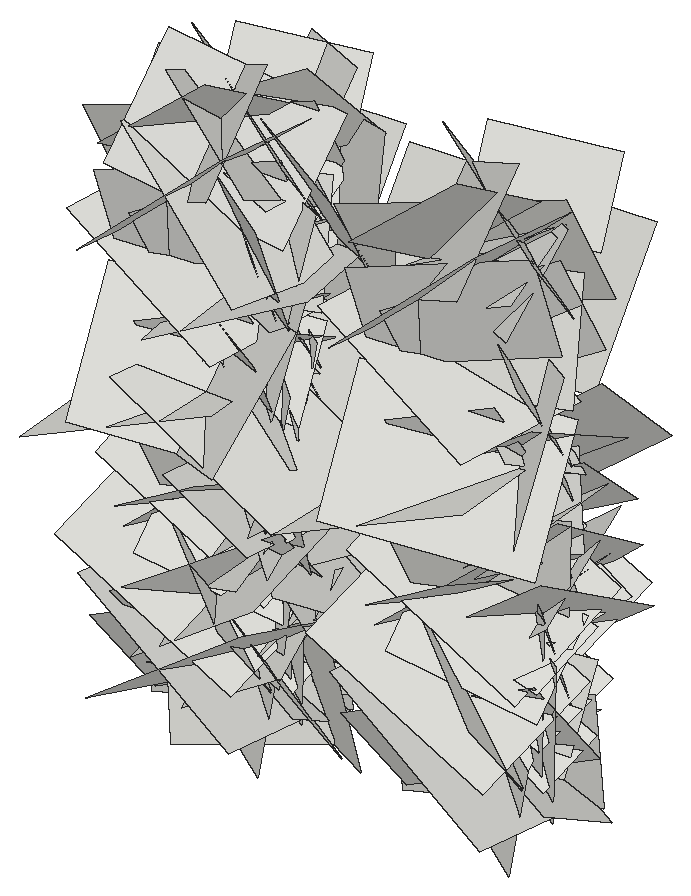
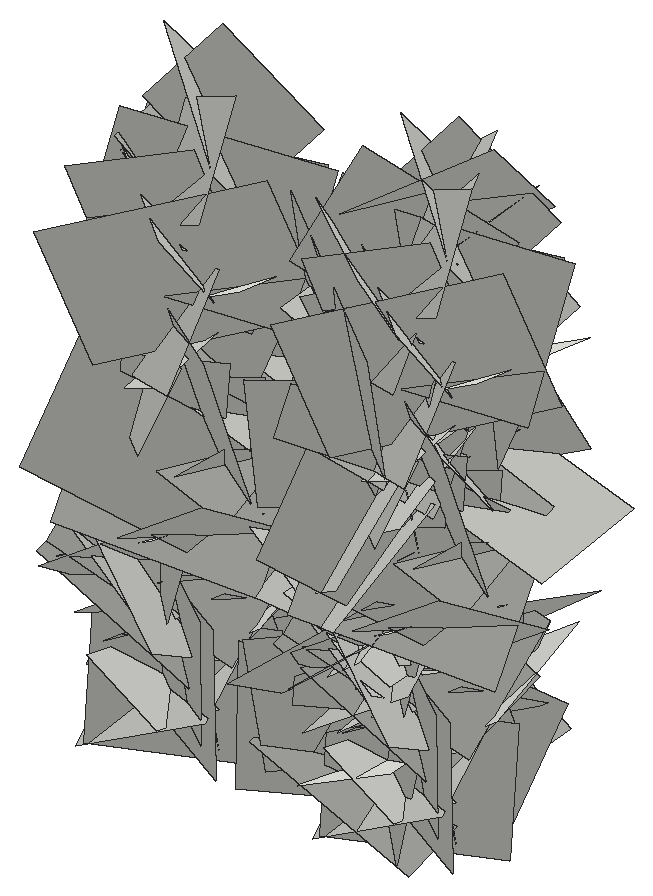
# SketchUp Ruby script. Lengths in inches.
U = 1.inch
M = Sketchup.active_model
def pt(a) = Geom::Point3d.new(a.map { |v| v * U })
def face(e, loops, mat)
  f = e.add_face(loops[0].map { |a| pt(a) })
  loops[1..].each { |l| e.add_face(l.map { |a| pt(a) }).erase! }
  f.material = f.back_material = mat if mat
  f
end
# faces: each face lists its corners as indices into pts; further lists are holes
def faces(e, pts, list, mat = nil) = list.each { |f| face(e, (f[0].is_a?(Array) ? f : [f]).map { |l| l.map { |i| pts[i] } }, mat) }
# xy, xz, yz: faces in a plane at the given z, y or x. An outline is a flat list of corners, or four numbers for a rectangle; further outlines are holes
def ring(l) = l.size == 4 ? [[l[0], l[1]], [l[2], l[1]], [l[2], l[3]], [l[0], l[3]]] : l.each_slice(2).to_a
def flat(e, list, mat, &to3) = list.each { |f| face(e, (f[0].is_a?(Array) ? f : [f]).map { |l| ring(l).map { |u, v| to3.(u, v) } }, mat) }
def xy(e, z, list, mat = nil) = flat(e, list, mat) { |x, y| [x, y, z] }
def xz(e, y, list, mat = nil) = flat(e, list, mat) { |x, z| [x, y, z] }
def yz(e, x, list, mat = nil) = flat(e, list, mat) { |y, z| [x, y, z] }
def lines(e, pts, list) = list.each { |a, b| e.add_line(pt(pts[a]), pt(pts[b])) }
# prism: a flat outline (further loops are holes) pulled along v
def prism(e, loops, v, mat = nil)
  f = face(e, loops, mat); d = Geom::Vector3d.new(v.map { |x| x * U })
  f.pushpull(f.normal.samedirection?(d) ? d.length : -d.length)
end
def box(e, o, s, mat = nil) = prism(e, [[o, [o[0] + s[0], o[1], o[2]], [o[0] + s[0], o[1] + s[1], o[2]], [o[0], o[1] + s[1], o[2]]]], [0, 0, s[2]], mat)
def at(x, y, z, deg = 0) = Geom::Transformation.translation(pt([x, y, z])) * Geom::Transformation.rotation(ORIGIN, Z_AXIS, deg.degrees)
def axes(o, x, y, z) = Geom::Transformation.new([*x, 0, *y, 0, *z, 0, *pt(o).to_a, 1])
def part(name) = M.definitions.add(name)
# library, detail: a bought-in or finely detailed component or shape, given as its bounding box
def library(name, o, s) = part(name).tap { |d| box(d.entities, o, s) }
def detail(e, o, s) = box(e.add_group.entities, o, s)
def put(e, d, t, mat = nil) = e.add_instance(d, t).tap { |i| i.material = mat if mat }
def group(e, t, mat = nil) = e.add_group.tap { |g| g.transformation = t; g.material = mat if mat }.entities
root = M.entities
c1 = part("Component\#6")
p = [[0.01,0,0],[0,3.24,4.54],[4.32,3.24,4.54],[4.33,0,0]]
faces(c1.entities,p,[[0,1,2,3]])
put(root,c1,axes([14.53,170.45,6.95],[-0.13562,-0.59571,0.16409],[0.06684,0.15411,0.60864],[0.65155,-0.13981,-0.02828]))
put(root,c1,axes([18.5,170.45,6.95],[0.13562,-0.59571,0.16409],[-0.06684,0.15411,0.60864],[-0.65155,-0.13981,-0.02828]))
put(root,c1,axes([24.34,170.45,6.95],[-0.13562,-0.59571,0.16409],[0.06684,0.15411,0.60864],[0.65155,-0.13981,-0.02828]))
put(root,c1,axes([18.5,172.51,13.7],[0.18405,-0.71312,-0.93832],[0.0125,-0.94735,0.72216],[-1.2492,-0.11455,-0.13102]))
put(root,c1,axes([14.53,172.51,13.7],[-0.18405,-0.71312,-0.93832],[-0.0125,-0.94735,0.72216],[1.2492,-0.11455,-0.13102]))
put(root,c1,axes([28.31,172.51,13.7],[0.18405,-0.71312,-0.93832],[0.0125,-0.94735,0.72216],[-1.2492,-0.11455,-0.13102]))
put(root,c1,axes([18.5,166.89,12.83],[-0.13197,1.26874,-0.04114],[-0.28106,-0.06642,-1.24587],[-1.31589,-0.11305,0.27023]))
put(root,c1,axes([14.53,166.89,12.83],[0.13197,1.26874,-0.04114],[0.28106,-0.06642,-1.24587],[1.31589,-0.11305,0.27023]))
put(root,c1,axes([28.31,166.89,12.83],[-0.13197,1.26874,-0.04114],[-0.28106,-0.06642,-1.24587],[-1.31589,-0.11305,0.27023]))
put(root,c1,axes([14.53,170.4375,18.81],[-0.19883,-0.70321,0.38228],[-0.06935,0.40479,0.71252],[0.84558,-0.13215,0.14832]))
put(root,c1,axes([18.5,170.4375,18.81],[0.19883,-0.70321,0.38228],[0.06935,0.40479,0.71252],[-0.84558,-0.13215,0.14832]))
put(root,c1,axes([24.34,170.4375,18.81],[-0.19883,-0.70321,0.38228],[-0.06935,0.40479,0.71252],[0.84558,-0.13215,0.14832]))
put(root,c1,axes([18.5,172.01,0.23],[0.18306,-1.21621,0.26629],[0.00588,0.26959,1.22768],[-1.31971,-0.16751,0.04241]))
put(root,c1,axes([14.53,172.01,0.23],[-0.18306,-1.21621,0.26629],[-0.00588,0.26959,1.22768],[1.31971,-0.16751,0.04241]))
put(root,c1,axes([28.31,172.01,0.23],[0.18306,-1.21621,0.26629],[0.00588,0.26959,1.22768],[-1.31971,-0.16751,0.04241]))
put(root,c1,axes([18.5,167.43,21.54],[-0.05686,1.16606,-0.16138],[0.18622,-0.15181,-1.15529],[-1.23383,-0.07665,-0.16693]))
put(root,c1,axes([14.53,167.43,21.54],[0.05686,1.16606,-0.16138],[-0.18622,-0.15181,-1.15529],[1.23383,-0.07665,-0.16693]))
put(root,c1,axes([28.31,167.43,21.54],[-0.05686,1.16606,-0.16138],[0.18622,-0.15181,-1.15529],[-1.23383,-0.07665,-0.16693]))
put(root,c1,axes([18.5,170.29,20.28],[-0.01759,0.35165,-0.94572],[-0.09141,-0.94289,-0.34909],[-1.06561,0.07508,0.04555]))
put(root,c1,axes([14.53,170.29,20.28],[0.01759,0.35165,-0.94572],[0.09141,-0.94289,-0.34909],[1.06561,0.07508,0.04555]))
put(root,c1,axes([28.31,170.29,20.28],[-0.01759,0.35165,-0.94572],[-0.09141,-0.94289,-0.34909],[-1.06561,0.07508,0.04555]))
put(root,c1,axes([18.5,166.61,20.4],[-0.01588,0.7114,0.79833],[0.18087,0.78977,-0.70057],[-1.11894,0.11757,-0.12458]))
put(root,c1,axes([14.53,166.61,20.4],[0.01588,0.7114,0.79833],[-0.18087,0.78977,-0.70057],[1.11894,0.11757,-0.12458]))
put(root,c1,axes([28.31,166.61,20.4],[-0.01588,0.7114,0.79833],[0.18087,0.78977,-0.70057],[-1.11894,0.11757,-0.12458]))
put(root,c1,axes([14.53,169.875,11.58],[-0.08121,-0.31714,0.54408],[0.11401,0.53345,0.32609],[0.65774,-0.13162,0.01065]))
put(root,c1,axes([18.5,169.875,11.58],[0.08121,-0.31714,0.54408],[-0.11401,0.53345,0.32609],[-0.65774,-0.13162,0.01065]))
put(root,c1,axes([24.34,169.875,11.58],[-0.08121,-0.31714,0.54408],[0.11401,0.53345,0.32609],[0.65774,-0.13162,0.01065]))
put(root,c1,axes([18.5,169.82,1.95],[0.02915,-0.64251,0.76006],[0.08177,0.75943,0.6392],[-1.05178,0.04123,0.07076]))
put(root,c1,axes([14.53,169.82,1.95],[-0.02915,-0.64251,0.76006],[-0.08177,0.75943,0.6392],[1.05178,0.04123,0.07076]))
put(root,c1,axes([28.31,169.82,1.95],[0.02915,-0.64251,0.76006],[0.08177,0.75943,0.6392],[-1.05178,0.04123,0.07076]))
put(root,c1,axes([18.5,173.1,4.27],[-0.006,-1.20261,-0.38975],[0.07836,-0.3894,1.20046],[-1.33775,-0.01742,0.07206]))
put(root,c1,axes([14.53,173.1,4.27],[0.006,-1.20261,-0.38975],[-0.07836,-0.3894,1.20046],[1.33775,-0.01742,0.07206]))
put(root,c1,axes([28.31,173.1,4.27],[-0.006,-1.20261,-0.38975],[0.07836,-0.3894,1.20046],[-1.33775,-0.01742,0.07206]))
put(root,c1,axes([14.53,169.57,7.53],[0.02893,-0.34038,0.60393],[-0.06424,0.60091,0.34142],[0.73203,0.06619,0.00609]))
put(root,c1,axes([18.5,169.57,7.53],[-0.02893,-0.34038,0.60393],[0.06424,0.60091,0.34142],[-0.73203,0.06619,0.00609]))
put(root,c1,axes([24.34,169.57,7.53],[0.02893,-0.34038,0.60393],[-0.06424,0.60091,0.34142],[0.73203,0.06619,0.00609]))
put(root,c1,axes([18.5,172.68,14.25],[-0.15371,-1.16437,-0.05617],[-0.14183,-0.0396,1.1664],[-1.22751,0.15038,-0.12774]))
put(root,c1,axes([14.53,172.68,14.25],[0.15371,-1.16437,-0.05617],[0.14183,-0.0396,1.1664],[1.22751,0.15038,-0.12774]))
put(root,c1,axes([28.31,172.68,14.25],[-0.15371,-1.16437,-0.05617],[-0.14183,-0.0396,1.1664],[-1.22751,0.15038,-0.12774]))
put(root,c1,axes([18.5,172.08,18.68],[0.05145,-0.65016,0.07549],[-0.09383,0.06848,0.64671],[-0.68743,-0.05801,-0.08262]))
put(root,c1,axes([14.53,172.08,18.68],[-0.05145,-0.65016,0.07549],[0.09383,0.06848,0.64671],[0.68743,-0.05801,-0.08262]))
put(root,c1,axes([24.34,172.08,18.68],[-0.05145,-0.65016,0.07549],[0.09383,0.06848,0.64671],[0.68743,-0.05801,-0.08262]))
put(root,c1,axes([14.53,168.08,6.15],[-0.10311,0.69666,0.5447],[-0.01855,0.54636,-0.70191],[0.9372,0.08746,0.04604]))
put(root,c1,axes([18.5,168.08,6.15],[0.10311,0.69666,0.5447],[0.01855,0.54636,-0.70191],[-0.9372,0.08746,0.04604]))
put(root,c1,axes([24.34,168.08,6.15],[-0.10311,0.69666,0.5447],[-0.01855,0.54636,-0.70191],[0.9372,0.08746,0.04604]))
put(root,c1,axes([18.5,170.37,5.28],[0.04044,0.69271,-0.86885],[-0.14808,-0.85947,-0.69137],[-1.16852,0.13289,0.05755]))
put(root,c1,axes([14.53,170.37,5.28],[-0.04044,0.69271,-0.86885],[0.14808,-0.85947,-0.69137],[1.16852,0.13289,0.05755]))
put(root,c1,axes([28.31,170.37,5.28],[0.04044,0.69271,-0.86885],[-0.14808,-0.85947,-0.69137],[-1.16852,0.13289,0.05755]))
put(root,c1,axes([18.5,171.61,19.65],[0.05512,0.44879,-0.89687],[0.12411,-0.89465,-0.44089],[-1.05579,-0.08174,-0.09865]))
put(root,c1,axes([14.53,171.61,19.65],[-0.05512,0.44879,-0.89687],[-0.12411,-0.89465,-0.44089],[1.05579,-0.08174,-0.09865]))
put(root,c1,axes([28.31,171.61,19.65],[0.05512,0.44879,-0.89687],[0.12411,-0.89465,-0.44089],[-1.05579,-0.08174,-0.09865]))
put(root,c1,axes([18.5,172.8125,18.6875],[0.10377,-0.25363,-0.96814],[-0.17625,-0.96337,0.23557],[-1.04612,0.13715,-0.13572]))
put(root,c1,axes([14.53,172.8125,18.6875],[-0.10377,-0.25363,-0.96814],[0.17625,-0.96337,0.23557],[1.04612,0.13715,-0.13572]))
put(root,c1,axes([28.31,172.8125,18.6875],[0.10377,-0.25363,-0.96814],[-0.17625,-0.96337,0.23557],[-1.04612,0.13715,-0.13572]))
put(root,c1,axes([18.5,173.43,2.26],[-0.13173,-0.86629,-0.47025],[0.00519,-0.47451,0.87284],[-1.04483,0.10686,0.06363]))
put(root,c1,axes([14.53,173.43,2.26],[0.13173,-0.86629,-0.47025],[-0.00519,-0.47451,0.87284],[1.04483,0.10686,0.06363]))
put(root,c1,axes([28.31,173.43,2.26],[-0.13173,-0.86629,-0.47025],[0.00519,-0.47451,0.87284],[-1.04483,0.10686,0.06363]))
put(root,c1,axes([14.53,172.62,2.82],[-0.11022,-0.07985,-0.84847],[0.01268,-0.85481,0.07898],[0.90326,0.00226,-0.10464]))
put(root,c1,axes([18.5,172.62,2.82],[0.11022,-0.07985,-0.84847],[-0.01268,-0.85481,0.07898],[-0.90326,0.00226,-0.10464]))
put(root,c1,axes([24.34,172.62,2.82],[-0.11022,-0.07985,-0.84847],[0.01268,-0.85481,0.07898],[0.90326,0.00226,-0.10464]))
put(root,c1,axes([18.5,172.18,10.26],[-0.13568,0.14362,-0.9313],[-0.0793,-0.93844,-0.13444],[-0.9957,0.05517,0.13761]))
put(root,c1,axes([28.31,172.18,10.26],[-0.13568,0.14362,-0.9313],[-0.0793,-0.93844,-0.13444],[-0.9957,0.05517,0.13761]))
put(root,c1,axes([14.53,172.18,10.26],[0.13568,0.14362,-0.9313],[0.0793,-0.93844,-0.13444],[0.9957,0.05517,0.13761]))
put(root,c1,axes([14.53,169.25,3.37],[-0.12984,0.58451,0.34416],[-0.01188,0.34794,-0.59491],[0.71891,0.11132,0.05233]))
put(root,c1,axes([18.5,169.25,3.37],[0.12984,0.58451,0.34416],[0.01188,0.34794,-0.59491],[-0.71891,0.11132,0.05233]))
put(root,c1,axes([24.34,169.25,3.37],[-0.12984,0.58451,0.34416],[-0.01188,0.34794,-0.59491],[0.71891,0.11132,0.05233]))
put(root,c1,axes([18.5,174.625,6.88],[-0.07025,-1.10898,-0.49527],[0.16839,-0.49966,1.09755],[-1.27636,-0.00489,0.17206]))
put(root,c1,axes([14.53,174.625,6.88],[0.07025,-1.10898,-0.49527],[-0.16839,-0.49966,1.09755],[1.27636,-0.00489,0.17206]))
put(root,c1,axes([28.31,174.625,6.88],[-0.07025,-1.10898,-0.49527],[0.16839,-0.49966,1.09755],[-1.27636,-0.00489,0.17206]))
put(root,c1,axes([18.5,173.47,4.9],[-0.07332,-0.2848,-0.87141],[0.0336,-0.87411,0.28317],[-0.9712,-0.00874,0.07558]))
put(root,c1,axes([14.53,173.47,4.9],[0.07332,-0.2848,-0.87141],[-0.0336,-0.87411,0.28317],[0.9712,-0.00874,0.07558]))
put(root,c1,axes([28.31,173.47,4.9],[-0.07332,-0.2848,-0.87141],[0.0336,-0.87411,0.28317],[-0.9712,-0.00874,0.07558]))
put(root,c1,axes([14.53,169.67,8.54],[-0.12628,0.08221,0.86907],[-0.11161,0.86937,-0.09667],[0.91857,0.11693,0.10773]))
put(root,c1,axes([18.5,169.67,8.54],[0.12628,0.08221,0.86907],[0.11161,0.86937,-0.09667],[-0.91857,0.11693,0.10773]))
put(root,c1,axes([24.34,169.67,8.54],[-0.12628,0.08221,0.86907],[-0.11161,0.86937,-0.09667],[0.91857,0.11693,0.10773]))
put(root,c1,axes([14.53,173.61,18.42],[0.00387,-0.64214,-0.38262],[0.01033,-0.38255,0.64212],[0.79227,0.00812,-0.0065]))
put(root,c1,axes([18.5,173.61,18.42],[-0.00387,-0.64214,-0.38262],[-0.01033,-0.38255,0.64212],[-0.79227,0.00812,-0.0065]))
put(root,c1,axes([24.34,173.61,18.42],[0.00387,-0.64214,-0.38262],[0.01033,-0.38255,0.64212],[0.79227,0.00812,-0.0065]))
put(root,c1,axes([18.5,173.47,6.03],[0.02519,-0.71274,-0.22366],[-0.1783,-0.22314,0.69319],[-0.7715,0.02829,-0.1675]))
put(root,c1,axes([14.53,173.47,6.03],[-0.02519,-0.71274,-0.22366],[0.1783,-0.22314,0.69319],[0.7715,0.02829,-0.1675]))
put(root,c1,axes([28.31,173.47,6.03],[0.02519,-0.71274,-0.22366],[-0.1783,-0.22314,0.69319],[-0.7715,0.02829,-0.1675]))
put(root,c1,axes([18.5,170.23,14.27],[0.02775,1.05616,-0.50439],[0.01222,-0.50473,-1.05626],[-1.24058,0.01865,-0.02169]))
put(root,c1,axes([14.53,170.23,14.27],[-0.02775,1.05616,-0.50439],[-0.01222,-0.50473,-1.05626],[1.24058,0.01865,-0.02169]))
put(root,c1,axes([28.31,170.23,14.27],[0.02775,1.05616,-0.50439],[0.01222,-0.50473,-1.05626],[-1.24058,0.01865,-0.02169]))
put(root,c1,axes([18.5,172.3,17.31],[0.17712,-0.66279,0.75583],[-0.05377,0.75967,0.67737],[-1.06423,-0.14869,0.09157]))
put(root,c1,axes([14.53,172.3,17.31],[-0.17712,-0.66279,0.75583],[0.05377,0.75967,0.67737],[1.06423,-0.14869,0.09157]))
put(root,c1,axes([28.31,172.3,17.31],[0.17712,-0.66279,0.75583],[-0.05377,0.75967,0.67737],[-1.06423,-0.14869,0.09157]))
put(root,c1,axes([18.5,171.9,21.66],[-0.05821,0.63814,-1.10333],[-0.23209,-1.09266,-0.62107],[-1.33097,0.16262,0.15656]))
put(root,c1,axes([14.53,171.9,21.66],[0.05821,0.63814,-1.10333],[0.23209,-1.09266,-0.62107],[1.33097,0.16262,0.15656]))
put(root,c1,axes([28.31,171.9,21.66],[-0.05821,0.63814,-1.10333],[-0.23209,-1.09266,-0.62107],[-1.33097,0.16262,0.15656]))
put(root,c1,axes([14.53,171.64,6.09],[-0.04085,-0.22846,0.61977],[0.06336,0.61707,0.23119],[0.6973,-0.06945,0.0153]))
put(root,c1,axes([18.5,171.64,6.09],[0.04085,-0.22846,0.61977],[-0.06336,0.61707,0.23119],[-0.6973,-0.06945,0.0153]))
put(root,c1,axes([24.34,171.64,6.09],[-0.04085,-0.22846,0.61977],[0.06336,0.61707,0.23119],[0.6973,-0.06945,0.0153]))
put(root,c1,axes([18.5,170.14,10.52],[-0.06349,0.95893,0.01002],[0.03302,0.01198,-0.96028],[-1.01599,-0.05954,-0.03183]))
put(root,c1,axes([14.53,170.14,10.52],[0.06349,0.95893,0.01002],[-0.03302,0.01198,-0.96028],[1.01599,-0.05954,-0.03183]))
put(root,c1,axes([28.31,170.14,10.52],[-0.06349,0.95893,0.01002],[0.03302,0.01198,-0.96028],[-1.01599,-0.05954,-0.03183]))
put(root,c1,axes([14.53,174.87,19.3],[-0.1513,-0.51657,-0.73784],[-0.06675,-0.7395,0.52991],[0.9524,-0.13389,-0.08008]))
put(root,c1,axes([18.5,174.87,19.3],[0.1513,-0.51657,-0.73784],[0.06675,-0.7395,0.52991],[-0.9524,-0.13389,-0.08008]))
put(root,c1,axes([24.34,174.87,19.3],[-0.1513,-0.51657,-0.73784],[-0.06675,-0.7395,0.52991],[0.9524,-0.13389,-0.08008]))
put(root,c1,axes([18.5,172.92,11.6],[-0.15777,-0.72106,0.34948],[0.01112,0.35368,0.73418],[-0.84929,0.13857,-0.05531]))
put(root,c1,axes([14.53,172.92,11.6],[0.15777,-0.72106,0.34948],[-0.01112,0.35368,0.73418],[0.84929,0.13857,-0.05531]))
put(root,c1,axes([28.31,172.92,11.6],[-0.15777,-0.72106,0.34948],[0.01112,0.35368,0.73418],[-0.84929,0.13857,-0.05531]))
put(root,c1,axes([18.5,169.35,10.4],[0.15861,0.37048,1.309],[-0.06067,1.31744,-0.36632],[-1.44077,-0.01469,0.15953]))
put(root,c1,axes([14.53,169.35,10.4],[-0.15861,0.37048,1.309],[0.06067,1.31744,-0.36632],[1.44077,-0.01469,0.15953]))
put(root,c1,axes([28.31,169.35,10.4],[0.15861,0.37048,1.309],[-0.06067,1.31744,-0.36632],[-1.44077,-0.01469,0.15953]))
put(root,c1,axes([18.5,171.5,10.51],[-0.09816,1.08592,-0.68794],[0.27584,-0.65961,-1.07622],[-1.33441,-0.21623,-0.17187]))
put(root,c1,axes([14.53,171.5,10.51],[0.09816,1.08592,-0.68794],[-0.27584,-0.65961,-1.07622],[1.33441,-0.21623,-0.17187]))
put(root,c1,axes([28.31,171.5,10.51],[-0.09816,1.08592,-0.68794],[0.27584,-0.65961,-1.07622],[-1.33441,-0.21623,-0.17187]))
put(root,c1,axes([18.5,170.67,8.7],[0.18467,1.04701,-0.56036],[0.0341,-0.57031,-1.0556],[-1.25832,0.1382,-0.11085]))
put(root,c1,axes([14.53,170.67,8.7],[-0.18467,1.04701,-0.56036],[-0.0341,-0.57031,-1.0556],[1.25832,0.1382,-0.11085]))
put(root,c1,axes([28.31,170.67,8.7],[0.18467,1.04701,-0.56036],[0.0341,-0.57031,-1.0556],[-1.25832,0.1382,-0.11085]))
put(root,c1,axes([18.5,174.22,3.89],[-0.08779,-0.72671,-0.31501],[-0.02258,-0.31457,0.73129],[-0.83927,0.08448,0.01327]))
put(root,c1,axes([14.53,174.22,3.89],[0.08779,-0.72671,-0.31501],[0.02258,-0.31457,0.73129],[0.83927,0.08448,0.01327]))
put(root,c1,axes([28.31,174.22,3.89],[-0.08779,-0.72671,-0.31501],[-0.02258,-0.31457,0.73129],[-0.83927,0.08448,0.01327]))
put(root,c1,axes([18.5,174.19,-1.125],[0.19779,-1.01545,0.55728],[-0.13113,0.54376,1.03224],[-1.22079,-0.22293,-0.02059]))
put(root,c1,axes([14.53,174.19,-1.125],[-0.19779,-1.01545,0.55728],[0.13113,0.54376,1.03224],[1.22079,-0.22293,-0.02059]))
put(root,c1,axes([28.31,174.19,-1.125],[0.19779,-1.01545,0.55728],[-0.13113,0.54376,1.03224],[-1.22079,-0.22293,-0.02059]))
put(root,c1,axes([14.53,171.41,10.85],[-0.07762,0.04197,0.59758],[0.0194,0.6019,-0.04003],[0.6347,-0.01326,0.07431]))
put(root,c1,axes([18.5,171.41,10.85],[0.07762,0.04197,0.59758],[-0.0194,0.6019,-0.04003],[-0.6347,-0.01326,0.07431]))
put(root,c1,axes([24.34,171.41,10.85],[-0.07762,0.04197,0.59758],[0.0194,0.6019,-0.04003],[0.6347,-0.01326,0.07431]))
put(root,c1,axes([18.5,173.32,3.72],[-0.0912,0.22313,-1.04907],[-0.17676,-1.04242,-0.20804],[-1.12306,0.14594,0.11794]))
put(root,c1,axes([14.53,173.32,3.72],[0.0912,0.22313,-1.04907],[0.17676,-1.04242,-0.20804],[1.12306,0.14594,0.11794]))
put(root,c1,axes([28.31,173.32,3.72],[-0.0912,0.22313,-1.04907],[-0.17676,-1.04242,-0.20804],[-1.12306,0.14594,0.11794]))
put(root,c1,axes([14.53,173.27,2.31],[0.02745,-0.60704,0.2793],[-0.09658,0.2737,0.6033],[0.70169,0.06142,0.07211]))
put(root,c1,axes([18.5,173.27,2.31],[-0.02745,-0.60704,0.2793],[0.09658,0.2737,0.6033],[-0.70169,0.06142,0.07211]))
put(root,c1,axes([24.34,173.27,2.31],[0.02745,-0.60704,0.2793],[-0.09658,0.2737,0.6033],[0.70169,0.06142,0.07211]))
put(root,c1,axes([18.5,172.23,12.17],[-0.04321,-0.56467,0.8488],[0.06772,0.84639,0.56613],[-1.07851,0.07577,0.00154]))
put(root,c1,axes([14.53,172.23,12.17],[0.04321,-0.56467,0.8488],[-0.06772,0.84639,0.56613],[1.07851,0.07577,0.00154]))
put(root,c1,axes([28.31,172.23,12.17],[-0.04321,-0.56467,0.8488],[0.06772,0.84639,0.56613],[-1.07851,0.07577,0.00154]))
put(root,c1,axes([18.5,170.77,1.94],[-0.10305,0.14958,1.1623],[0.03,1.16625,-0.14772],[-1.24184,0.01576,-0.10002]))
put(root,c1,axes([14.53,170.77,1.94],[0.10305,0.14958,1.1623],[-0.03,1.16625,-0.14772],[1.24184,0.01576,-0.10002]))
put(root,c1,axes([28.31,170.77,1.94],[-0.10305,0.14958,1.1623],[0.03,1.16625,-0.14772],[-1.24184,0.01576,-0.10002]))
put(root,c1,axes([18.5,172.28,10.96],[-0.19399,-0.26613,0.68464],[0.06344,0.69782,0.28725],[-0.77602,0.12358,-0.14766]))
put(root,c1,axes([14.53,172.28,10.96],[0.19399,-0.26613,0.68464],[-0.06344,0.69782,0.28725],[0.77602,0.12358,-0.14766]))
put(root,c1,axes([28.31,172.28,10.96],[-0.19399,-0.26613,0.68464],[0.06344,0.69782,0.28725],[-0.77602,0.12358,-0.14766]))
put(root,c1,axes([18.5,172.17,3.88],[-0.10658,-0.21665,0.83392],[0.00523,0.83942,0.21867],[-0.91328,0.03009,-0.09606]))
put(root,c1,axes([14.53,172.17,3.88],[0.10658,-0.21665,0.83392],[-0.00523,0.83942,0.21867],[0.91328,0.03009,-0.09606]))
put(root,c1,axes([28.31,172.17,3.88],[-0.10658,-0.21665,0.83392],[0.00523,0.83942,0.21867],[-0.91328,0.03009,-0.09606]))
put(root,c1,axes([18.5,172.79,12.08],[-0.24348,0.91998,-0.78066],[-0.03668,-0.79938,-0.93185],[-1.27843,-0.15228,0.17542]))
put(root,c1,axes([14.53,172.79,12.08],[0.24348,0.91998,-0.78066],[0.03668,-0.79938,-0.93185],[1.27843,-0.15228,0.17542]))
put(root,c1,axes([28.31,172.79,12.08],[-0.24348,0.91998,-0.78066],[-0.03668,-0.79938,-0.93185],[-1.27843,-0.15228,0.17542]))
put(root,c1,axes([18.5,171.28,0.09],[0.0277,-0.00252,1.28462],[-0.09278,1.2819,0.0043],[-1.35854,-0.08759,0.0259]))
put(root,c1,axes([28.31,171.28,0.09],[0.0277,-0.00252,1.28462],[-0.09278,1.2819,0.0043],[-1.35854,-0.08759,0.0259]))
put(root,c1,axes([14.53,171.28,0.09],[-0.0277,-0.00252,1.28462],[0.09278,1.2819,0.0043],[1.35854,-0.08759,0.0259]))
put(root,c1,axes([14.53,174.97,1.18],[-0.10067,-0.62121,-0.06126],[0.13552,-0.08001,0.61313],[0.64765,-0.07982,-0.13782]))
put(root,c1,axes([18.5,174.97,1.18],[0.10067,-0.62121,-0.06126],[-0.13552,-0.08001,0.61313],[-0.64765,-0.07982,-0.13782]))
put(root,c1,axes([24.34,174.97,1.18],[-0.10067,-0.62121,-0.06126],[0.13552,-0.08001,0.61313],[0.64765,-0.07982,-0.13782]))
put(root,c1,axes([18.5,176.36,18.92],[-0.19548,-0.4632,-1.27504],[0.04093,-1.28804,0.46234],[-1.43738,0.02631,0.18657]))
put(root,c1,axes([14.53,176.36,18.92],[0.19548,-0.4632,-1.27504],[-0.04093,-1.28804,0.46234],[1.43738,0.02631,0.18657]))
put(root,c1,axes([28.31,176.36,18.92],[-0.19548,-0.4632,-1.27504],[0.04093,-1.28804,0.46234],[-1.43738,0.02631,0.18657]))
put(root,c1,axes([18.5,176.11,6.43],[-0.23133,-1.0261,-0.61864],[-0.04368,-0.62202,1.04624],[-1.2693,0.20842,0.07674]))
put(root,c1,axes([14.53,176.11,6.43],[0.23133,-1.0261,-0.61864],[0.04368,-0.62202,1.04624],[1.2693,0.20842,0.07674]))
put(root,c1,axes([28.31,176.11,6.43],[-0.23133,-1.0261,-0.61864],[-0.04368,-0.62202,1.04624],[-1.2693,0.20842,0.07674]))
put(root,c1,axes([18.5,175.17,6.35],[-0.11089,-0.78923,-0.08985],[-0.10937,-0.07636,0.79084],[-0.83485,0.11483,-0.09167]))
put(root,c1,axes([14.53,175.17,6.35],[0.11089,-0.78923,-0.08985],[0.10937,-0.07636,0.79084],[0.83485,0.11483,-0.09167]))
put(root,c1,axes([28.31,175.17,6.35],[-0.11089,-0.78923,-0.08985],[-0.10937,-0.07636,0.79084],[-0.83485,0.11483,-0.09167]))
put(root,c1,axes([14.53,175.4,4.97],[0.01432,-0.74639,-0.04739],[-0.08616,-0.04858,0.74199],[0.78807,0.00825,0.08199]))
put(root,c1,axes([18.5,175.4,4.97],[-0.01432,-0.74639,-0.04739],[0.08616,-0.04858,0.74199],[-0.78807,0.00825,0.08199]))
put(root,c1,axes([24.34,175.4,4.97],[0.01432,-0.74639,-0.04739],[-0.08616,-0.04858,0.74199],[0.78807,0.00825,0.08199]))
put(root,c1,axes([18.5,173.68,14.42],[-0.07839,0.88361,-0.83437],[0.27617,-0.80495,-0.87555],[-1.25826,-0.23172,-0.14019]))
put(root,c1,axes([14.53,173.68,14.42],[0.07839,0.88361,-0.83437],[-0.27617,-0.80495,-0.87555],[1.25826,-0.23172,-0.14019]))
put(root,c1,axes([28.31,173.68,14.42],[-0.07839,0.88361,-0.83437],[0.27617,-0.80495,-0.87555],[-1.25826,-0.23172,-0.14019]))
put(root,c1,axes([14.53,171.94,19.49],[-0.08782,0.36838,0.63269],[0.00702,0.63708,-0.37006],[0.77601,0.03592,0.07495]))
put(root,c1,axes([18.5,171.94,19.49],[0.08782,0.36838,0.63269],[-0.00702,0.63708,-0.37006],[-0.77601,0.03592,0.07495]))
put(root,c1,axes([24.34,171.94,19.49],[-0.08782,0.36838,0.63269],[0.00702,0.63708,-0.37006],[0.77601,0.03592,0.07495]))
put(root,c1,axes([18.5,170.9375,7.01],[-0.11124,0.9843,0.53665],[0.15751,0.54645,-0.97322],[-1.17787,-0.01989,-0.18083]))
put(root,c1,axes([14.53,170.9375,7.01],[0.11124,0.9843,0.53665],[-0.15751,0.54645,-0.97322],[1.17787,-0.01989,-0.18083]))
put(root,c1,axes([28.31,170.9375,7.01],[-0.11124,0.9843,0.53665],[0.15751,0.54645,-0.97322],[-1.17787,-0.01989,-0.18083]))
